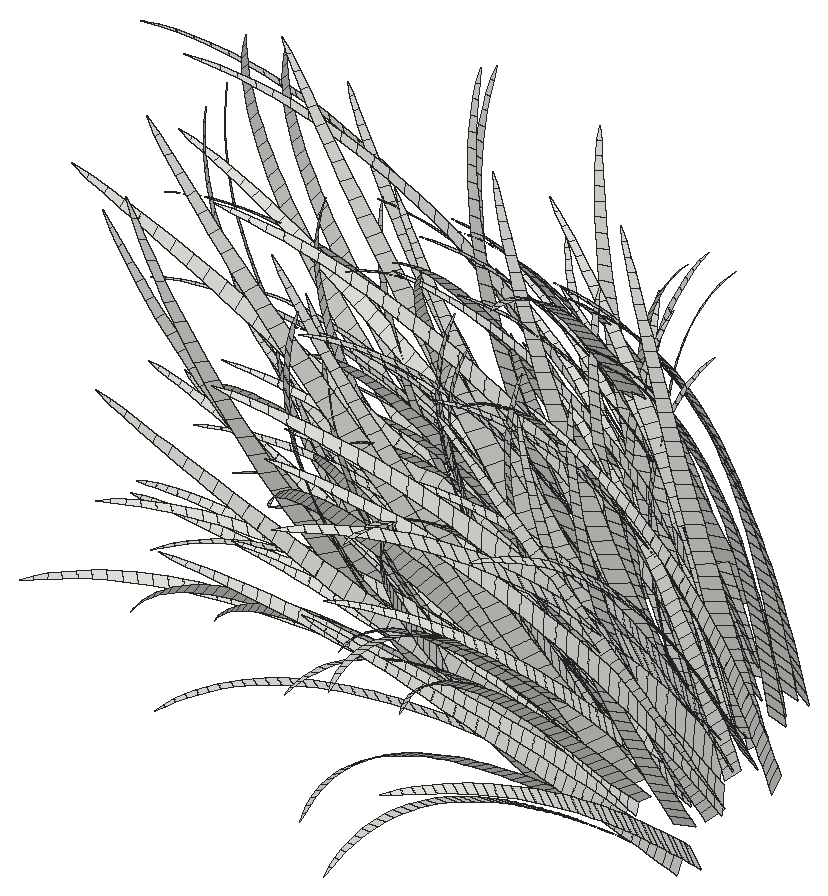
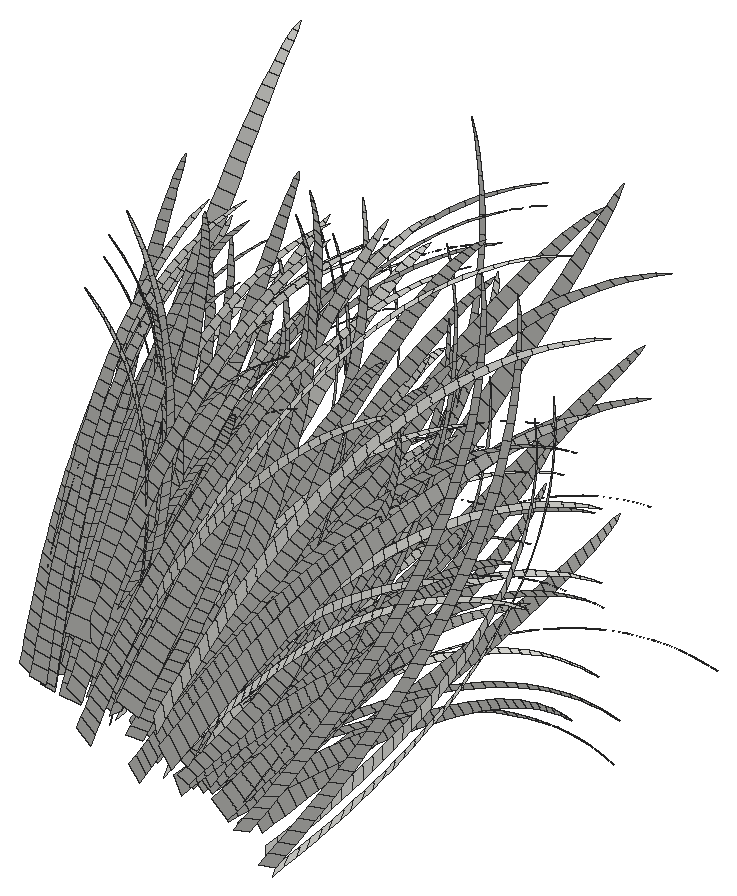
# SketchUp Ruby script. Lengths in inches.
U = 1.inch
M = Sketchup.active_model
def pt(a) = Geom::Point3d.new(a.map { |v| v * U })
def face(e, loops, mat)
  f = e.add_face(loops[0].map { |a| pt(a) })
  loops[1..].each { |l| e.add_face(l.map { |a| pt(a) }).erase! }
  f.material = f.back_material = mat if mat
  f
end
# faces: each face lists its corners as indices into pts; further lists are holes
def faces(e, pts, list, mat = nil) = list.each { |f| face(e, (f[0].is_a?(Array) ? f : [f]).map { |l| l.map { |i| pts[i] } }, mat) }
# xy, xz, yz: faces in a plane at the given z, y or x. An outline is a flat list of corners, or four numbers for a rectangle; further outlines are holes
def ring(l) = l.size == 4 ? [[l[0], l[1]], [l[2], l[1]], [l[2], l[3]], [l[0], l[3]]] : l.each_slice(2).to_a
def flat(e, list, mat, &to3) = list.each { |f| face(e, (f[0].is_a?(Array) ? f : [f]).map { |l| ring(l).map { |u, v| to3.(u, v) } }, mat) }
def xy(e, z, list, mat = nil) = flat(e, list, mat) { |x, y| [x, y, z] }
def xz(e, y, list, mat = nil) = flat(e, list, mat) { |x, z| [x, y, z] }
def yz(e, x, list, mat = nil) = flat(e, list, mat) { |y, z| [x, y, z] }
def lines(e, pts, list) = list.each { |a, b| e.add_line(pt(pts[a]), pt(pts[b])) }
# prism: a flat outline (further loops are holes) pulled along v
def prism(e, loops, v, mat = nil)
  f = face(e, loops, mat); d = Geom::Vector3d.new(v.map { |x| x * U })
  f.pushpull(f.normal.samedirection?(d) ? d.length : -d.length)
end
def box(e, o, s, mat = nil) = prism(e, [[o, [o[0] + s[0], o[1], o[2]], [o[0] + s[0], o[1] + s[1], o[2]], [o[0], o[1] + s[1], o[2]]]], [0, 0, s[2]], mat)
def at(x, y, z, deg = 0) = Geom::Transformation.translation(pt([x, y, z])) * Geom::Transformation.rotation(ORIGIN, Z_AXIS, deg.degrees)
def axes(o, x, y, z) = Geom::Transformation.new([*x, 0, *y, 0, *z, 0, *pt(o).to_a, 1])
def part(name) = M.definitions.add(name)
# library, detail: a bought-in or finely detailed component or shape, given as its bounding box
def library(name, o, s) = part(name).tap { |d| box(d.entities, o, s) }
def detail(e, o, s) = box(e.add_group.entities, o, s)
def put(e, d, t, mat = nil) = e.add_instance(d, t).tap { |i| i.material = mat if mat }
def group(e, t, mat = nil) = e.add_group.tap { |g| g.transformation = t; g.material = mat if mat }.entities
root = M.entities
c1 = part("fur_instance\#8")
p = [[-0.25,1.49,0.03],[0.25,-1.49,-0.03],[0.44,-1.47,1.51],[-0.05,1.47,1.57],[0.65,-1.44,3.05],[0.16,1.45,3.11],
  [0.86,-1.42,4.59],[0.38,1.44,4.65],[1.1,-1.39,6.13],[0.62,1.43,6.18],[1.34,-1.35,7.66],[0.875,1.42,7.72],
  [1.6,-1.32,9.19],[1.14,1.41,9.25],[1.88,-1.28,10.72],[1.43,1.41,10.78],[2.18,-1.24,12.25],[1.73,1.41,12.3],
  [2.49,-1.19,13.77],[2.05,1.41,13.82],[2.83,-1.15,15.29],[2.4,1.41,15.34],[3.18,-1.09,16.8],[2.76,1.42,16.85],
  [3.56,-1.03,18.31],[3.14,1.43,18.35],[3.96,-0.97,19.81],[3.55,1.44,19.85],[4.38,-0.91,21.3],[3.99,1.46,21.35],
  [4.84,-0.83,22.78],[4.45,1.48,22.83],[5.32,-0.76,24.26],[4.93,1.51,24.31],[5.82,-0.67,25.73],[5.45,1.54,25.77],
  [6.36,-0.59,27.18],[6,1.57,27.23],[6.93,-0.49,28.625],[6.58,1.61,28.67],[7.54,-0.39,30.05],[7.19,1.66,30.1],
  [8.18,-0.28,31.47],[7.84,1.71,31.51],[8.85,-0.16,32.86],[8.53,1.77,32.9],[9.57,-0.04,34.24],[9.25,1.83,34.27],
  [10.32,0.09,35.59],[10.02,1.9,35.625],[11.12,0.23,36.92],[10.82,1.97,36.95],[11.95,0.38,38.22],[11.67,2.06,38.25],
  [12.84,0.54,39.49],[12.57,2.14,39.52],[13.76,0.71,40.73],[13.51,2.24,40.76],[14.73,0.89,41.93],[14.49,2.34,41.95],
  [15.75,1.08,43.09],[15.52,2.45,43.11],[16.82,1.28,44.2],[16.6,2.5625,44.23],[17.93,1.5,45.27],[17.73,2.68,45.29],
  [19.08,1.73,46.28],[18.9,2.81,46.3],[20.29,1.97,47.24],[20.125,2.93,47.26],[21.53,2.22,48.13],[21.39,3.0625,48.15],
  [22.82,2.5,48.96],[22.7,3.1875,48.98],[24.14,2.8125,49.72],[24.06,3.3,49.73],[25.48,3.27,50.41]]
faces(c1.entities,p,[[0,1,2,3],[3,2,4,5],[5,4,6,7],[7,6,8,9],[9,8,10,11],[11,10,12,13],[13,12,14,15],[15,14,16,17],
  [17,16,18,19],[19,18,20,21],[21,20,22,23],[23,22,24,25],[25,24,26,27],[27,26,28,29],[29,28,30,31],[31,30,32,33],
  [33,32,34,35],[35,34,36,37],[37,36,38,39],[39,38,40,41],[41,40,42,43],[43,42,44,45],[45,44,46,47],[47,46,48,49],
  [49,48,50,51],[51,50,52,53],[53,52,54,55],[55,54,56,57],[57,56,58,59],[59,58,60,61],[61,60,62,63],[63,62,64,65],
  [65,64,66,67],[67,66,68,69],[69,68,70,71],[71,70,72,73],[73,72,74,75],[75,74,76]])
put(root,c1,axes([286.59,30.47,9.65],[0.27343,-0.05373,0.34841],[-0.11723,0.29702,0.06467],[-0.32726,-0.11352,0.28294]))
put(root,c1,axes([287.23,30.26,10.09],[0.23007,0.02662,0.34929],[-0.18351,0.2974,-0.02967],[-0.32374,-0.1123,0.27989]))
put(root,c1,axes([285.25,32.66,11.29],[0.334,-0.2152,0.2493],[0.13177,0.25584,0.18399],[-0.3051,-0.07912,0.37064]))
put(root,c1,axes([291.09,32.8125,16.03],[-0.40111,-0.111,-0.15079],[0.2354,-0.31959,0.01115],[-0.14507,-0.1083,0.47608]))
put(root,c1,axes([291.52,27.75,9.48],[-0.20253,0.22492,-0.01123],[-0.17196,-0.03802,-0.28818],[-0.24112,-0.12808,0.22836]))
put(root,c1,axes([292.69,26.93,10.13],[-0.26498,0.16022,-0.17783],[-0.02095,-0.16252,-0.22723],[-0.24124,-0.12814,0.22846]))
put(root,c1,axes([287.03,32.11,12.13],[0.3301,-0.20151,0.24919],[0.11757,0.2566,0.17128],[-0.29775,-0.07722,0.36172]))
put(root,c1,axes([291.21,31.99,14.07],[-0.17529,-0.2316,-0.142],[0.33875,-0.20497,0.16137],[-0.21428,-0.07814,0.39369]))
put(root,c1,axes([292.88,25.97,10.52],[-0.32801,0.05137,-0.26925],[0.18585,-0.20887,-0.21385],[-0.19763,-0.22375,0.26878]))
put(root,c1,axes([292.88,26.65,9.85],[-0.28984,0.15344,-0.12784],[-0.02507,-0.13644,-0.25763],[-0.20658,-0.15978,0.2261]))
put(root,c1,axes([293.18,28.9,13.9],[-0.37766,0.184,-0.06914],[-0.15358,-0.20823,-0.20885],[-0.16081,-0.1578,0.39181]))
put(root,c1,axes([292.93,26.43,10.32],[-0.31045,0.17685,-0.06933],[-0.11896,-0.14445,-0.24345],[-0.18306,-0.15633,0.29554]))
put(root,c1,axes([292.82,29.91,11.98],[-0.30983,-0.00394,-0.17456],[0.06503,-0.26267,0.03289],[-0.18102,-0.0412,0.32902]))
put(root,c1,axes([292.9,29.58,13.37],[-0.30671,-0.07302,-0.20131],[0.19117,-0.27097,0.01937],[-0.18997,-0.09935,0.36653]))
put(root,c1,axes([291.91,26.05,10.63],[-0.20515,0.19921,0.286],[-0.39464,0.04212,-0.25253],[-0.15677,-0.2771,0.29704]))
put(root,c1,axes([290.35,29.43,10.8],[0.11044,-0.26664,-0.03562],[0.2879,-0.01439,0.25595],[-0.24023,-0.09964,0.30634]))
put(root,c1,axes([293.35,26.83,10.48],[-0.21721,0.20602,0.03558],[-0.22128,-0.05396,-0.23339],[-0.17073,-0.1458,0.27564]))
put(root,c1,axes([294.49,26.96,13.81],[-0.4809,0.15467,0.07003],[-0.17758,-0.1848,-0.34168],[-0.0839,-0.29221,0.4025]))
put(root,c1,axes([292.82,27.34,10.21],[-0.12157,0.22306,0.06553],[-0.25945,0.01126,-0.21995],[-0.19306,-0.11653,0.26984]))
put(root,c1,axes([290.16,27.27,9.43],[0.16873,-0.23329,-0.16268],[0.2954,-0.05676,0.29434],[-0.24156,-0.18683,0.26439]))
put(root,c1,axes([294.54,30.98,16.64],[-0.45841,-0.0448,-0.1227],[0.16046,-0.32039,-0.10023],[-0.09604,-0.16019,0.48225]))
put(root,c1,axes([293.29,28.56,10.54],[-0.11106,-0.1633,-0.14192],[0.22222,-0.16383,0.16068],[-0.2111,-0.05474,0.25645]))
put(root,c1,axes([294.5,25.83,11.2],[-0.36489,0.00046,-0.19285],[0.17529,-0.2126,-0.2068],[-0.11798,-0.22209,0.32702]))
put(root,c1,axes([293.99,26.59,11.08],[-0.20712,-0.07699,-0.24552],[0.24774,-0.208,-0.01302],[-0.1778,-0.15184,0.28705]))
put(root,c1,axes([293.27,28.91,13.42],[-0.15645,0.26226,0.09015],[-0.35289,-0.02097,-0.18778],[-0.15226,-0.14941,0.37098]))
put(root,c1,axes([294.61,29.11,11.65],[-0.25641,-0.05967,-0.14526],[0.12307,-0.22834,0.06607],[-0.16263,-0.03702,0.2956]))
put(root,c1,axes([293.88,25.64,11.62],[-0.31647,0.23033,0.24139],[-0.40723,-0.07569,-0.25469],[-0.08441,-0.29398,0.40494]))
put(root,c1,axes([290.57,27.84,9.43],[0.27393,-0.09989,0.26383],[-0.07841,0.22332,0.16142],[-0.25859,-0.13736,0.2449]))
put(root,c1,axes([294.43,26.1,10.01],[-0.20297,0.18888,0.02954],[-0.20068,-0.0525,-0.2153],[-0.15716,-0.13421,0.25373]))
put(root,c1,axes([294,25.73,9.63],[-0.1796,-0.03718,-0.28054],[0.25918,-0.17602,-0.0633],[-0.1653,-0.18714,0.2248]))
put(root,c1,axes([295.09,25.85,10.55],[-0.31089,0.06016,-0.13906],[0.05838,-0.17982,-0.18276],[-0.13322,-0.16333,0.26664]))
put(root,c1,axes([289.54,28.61,11.13],[0.35824,-0.10563,0.23396],[-0.03698,0.2601,0.16876],[-0.24267,-0.14648,0.33917]))
put(root,c1,axes([292.97,24.9375,9.61],[-0.15927,0.19141,0.39707],[-0.5038,0.04411,-0.1792],[-0.10137,-0.33957,0.3384]))
put(root,c1,axes([295.47,24.97,10.55],[-0.40671,0.13906,0.11983],[-0.19446,-0.09353,-0.35183],[-0.08649,-0.28972,0.28872]))
put(root,c1,axes([292.35,27.91,11],[0.09607,0.16636,0.21346],[-0.29279,0.17326,-0.12392],[-0.20763,-0.12533,0.2902]))
put(root,c1,axes([294.18,27.19,13.6],[-0.24749,0.26545,0.14907],[-0.39506,-0.07422,-0.19021],[-0.10328,-0.2127,0.42576]))
put(root,c1,axes([294.73,26.92,12.03],[-0.31144,-0.04433,-0.1638],[0.17873,-0.22297,-0.09563],[-0.11163,-0.15329,0.33567]))
put(root,c1,axes([294.97,26.6,11.01],[-0.16359,0.19718,0.06974],[-0.23715,-0.01659,-0.20797],[-0.15863,-0.13546,0.2561]))
put(root,c1,axes([294.36,30.1,11.41],[-0.13255,-0.19412,-0.04324],[0.25386,-0.13806,0.15203],[-0.15874,-0.01602,0.29618]))
put(root,c1,axes([293.23,27.37,10.11],[0.05622,-0.22028,-0.06146],[0.25349,-0.04511,0.20874],[-0.20228,-0.0839,0.25794]))
put(root,c1,axes([291.99,26.66,9.55],[0.19826,-0.21945,-0.10113],[0.24048,-0.01499,0.29104],[-0.22131,-0.17117,0.24222]))
put(root,c1,axes([295.96,26.78,12.57],[-0.37408,0.03214,-0.09204],[0.05374,-0.22112,-0.17294],[-0.08373,-0.17243,0.34515]))
put(root,c1,axes([292.83,28.6,10.86],[0.14214,-0.23634,0.06971],[0.22005,0.06034,0.21505],[-0.2226,-0.05773,0.27043]))
put(root,c1,axes([292.76,29.2,12.34],[0.06163,-0.26061,-0.05185],[0.33201,-0.02894,0.18171],[-0.1775,-0.09282,0.34246]))
put(root,c1,axes([296.13,24.84,10.15],[-0.38075,0.07768,-0.02207],[-0.01808,-0.11852,-0.3135],[-0.07313,-0.24497,0.24413]))
put(root,c1,axes([295.55,28.38,12.91],[-0.29669,-0.08119,-0.1125],[0.1791,-0.23152,-0.01214],[-0.09804,-0.09366,0.35151]))
put(root,c1,axes([294.97,25.4,9.79],[-0.08632,0.15484,0.21721],[-0.29175,0.07846,-0.1727],[-0.1595,-0.18058,0.21691]))
put(root,c1,axes([296.28,30.79,13.71],[-0.31442,-0.10008,-0.0717],[0.17027,-0.25235,0.08233],[-0.10906,-0.0245,0.3674]))
put(root,c1,axes([294.48,28.84,11.72],[-0.04846,-0.21474,-0.06537],[0.28534,-0.09466,0.14944],[-0.1626,-0.0593,0.29875]))
put(root,c1,axes([296.46,25.04,10.21],[-0.31964,0.05744,-0.08852],[0.03295,-0.15868,-0.20626],[-0.09365,-0.17629,0.25958]))
put(root,c1,axes([296.53,26.36,11.67],[-0.31367,0.05166,-0.09146],[0.01951,-0.19214,-0.13854],[-0.0977,-0.13416,0.29378]))
put(root,c1,axes([294.97,28.29,12.09],[-0.06107,-0.20437,-0.10373],[0.29349,-0.11146,0.13184],[-0.15758,-0.08241,0.30403]))
put(root,c1,axes([292.65,27.21,10.55],[0.22564,-0.22209,0.02694],[0.20271,0.08113,0.24146],[-0.20438,-0.12337,0.28566]))
put(root,c1,axes([295.73,27.23,12.77],[-0.1569,0.2286,0.10904],[-0.32818,-0.02785,-0.15821],[-0.11309,-0.15528,0.34003]))
put(root,c1,axes([297.22,28.28,15.37],[-0.48448,0.00048,-0.04012],[0.07209,-0.2662,-0.24534],[-0.01781,-0.23845,0.43674]))
put(root,c1,axes([293.88,25.5,9.7],[0.14772,0.06981,0.31071],[-0.30774,0.18182,0.01975],[-0.17895,-0.2026,0.24337]))
put(root,c1,axes([296.17,25.125,10.97],[-0.24536,0.19524,0.21246],[-0.35336,-0.05273,-0.20133],[-0.07041,-0.24522,0.33777]))
put(root,c1,axes([295.57,27.91,12.12],[-0.06025,-0.19978,-0.10172],[0.28707,-0.10941,0.12883],[-0.15419,-0.08063,0.29748]))
put(root,c1,axes([291.96,26.95,11.7],[0.27785,-0.24567,-0.11356],[0.31431,0.05376,0.28262],[-0.17668,-0.21661,0.35363]))
put(root,c1,axes([293.34,28.62,13.62],[0.18292,0.18783,0.21033],[-0.35625,0.19804,-0.04959],[-0.15796,-0.15501,0.38486]))
put(root,c1,axes([295.89,31.56,13.24],[-0.16074,-0.22509,0.01009],[0.31616,-0.14511,0.10525],[-0.09686,-0.01193,0.36183]))
put(root,c1,axes([292.11,29.1,12.95],[0.32177,-0.21274,0.07133],[0.19821,0.17649,0.19557],[-0.17683,-0.12709,0.37373]))
put(root,c1,axes([291.88,25.43,9.8],[0.36191,0.00675,0.33836],[-0.31641,0.21997,0.23571],[-0.16944,-0.29949,0.32104]))
put(root,c1,axes([294.33,27.9,13.69],[0.10522,0.22276,0.21396],[-0.40669,0.14528,-0.0588],[-0.1306,-0.17932,0.39268]))
put(root,c1,axes([295.03,27.92,12.46],[0.04713,-0.23319,-0.08917],[0.32063,-0.04249,0.15465],[-0.15163,-0.10898,0.32048]))
put(root,c1,axes([295.61,30.37,15.29],[-0.09495,-0.26399,-0.12104],[0.41267,-0.12196,0.06705],[-0.10338,-0.12826,0.42496]))
put(root,c1,axes([294.625,30.24,14.41],[0.02749,-0.28529,-0.04854],[0.39441,-0.03638,0.11901],[-0.12332,-0.09206,0.40471]))
put(root,c1,axes([293.7,27.38,10.89],[0.2739,-0.05108,0.20185],[-0.0714,0.21464,0.10324],[-0.19072,-0.11512,0.26657]))
put(root,c1,axes([296.78,27.66,13.94],[-0.30159,-0.14954,-0.10961],[0.28485,-0.21676,-0.0779],[-0.03755,-0.15132,0.40536]))
put(root,c1,axes([295.99,25.24,10.68],[-0.01763,-0.16784,-0.246],[0.36343,-0.09136,0.06391],[-0.10604,-0.19963,0.29394]))
put(root,c1,axes([293.74,26.66,11.29],[0.29218,0.02035,0.226],[-0.20172,0.21186,0.12397],[-0.14953,-0.18332,0.29929]))
put(root,c1,axes([298.23,27.93,12.79],[-0.30076,0.11654,-0.01023],[-0.13091,-0.19765,-0.03854],[-0.03233,-0.07151,0.33559]))
put(root,c1,axes([295.5,25.92,10.87],[0.0874,-0.18327,-0.1671],[0.30131,-0.04217,0.15478],[-0.13212,-0.16199,0.26446]))
put(root,c1,axes([297.23,28.02,12.74],[-0.08042,0.22658,0.04044],[-0.31016,-0.01086,-0.09649],[-0.09064,-0.0866,0.32499]))
put(root,c1,axes([297.87,30.0625,14.61],[-0.28554,-0.16794,-0.04721],[0.27744,-0.2201,-0.01414],[-0.03336,-0.09063,0.40665]))
put(root,c1,axes([297.125,30.625,14.38],[-0.18942,-0.22658,-0.02013],[0.33953,-0.1634,0.03397],[-0.04803,-0.05962,0.39971]))
put(root,c1,axes([295.45,28.78,12.12],[0.18989,-0.20261,0.10406],[0.21185,0.12115,0.12104],[-0.16267,-0.03703,0.29567]))
put(root,c1,axes([295.74,24.72,9.42],[0.0858,-0.14547,-0.26588],[0.34076,-0.06868,0.14201],[-0.12385,-0.21892,0.23467]))
put(root,c1,axes([294.01,26.75,11.5],[0.32008,-0.01898,0.19642],[-0.14214,0.20908,0.16147],[-0.14749,-0.18083,0.29522]))
put(root,c1,axes([298.91,28.66,14.45],[-0.38324,-0.06278,-0.0243],[0.13399,-0.24652,-0.1286],[0.00956,-0.15154,0.39527]))
put(root,c1,axes([298.92,28.0625,13.11],[-0.32632,0.09549,0.01183],[-0.10602,-0.21576,-0.04162],[-0.01005,-0.0835,0.34927]))
put(root,c1,axes([299.78,25.77,12.74],[-0.51625,-0.01769,0.01101],[0.05539,-0.22677,-0.34952],[0.04511,-0.30441,0.40404]))
put(root,c1,axes([298.68,25.23,11.32],[-0.31274,-0.0305,-0.0904],[0.13256,-0.1462,-0.20962],[-0.01285,-0.1978,0.26335]))
put(root,c1,axes([299.29,24.02,9.18],[-0.33771,0.05415,0.06448],[-0.07902,-0.09732,-0.27357],[-0.01313,-0.22725,0.21826]))
put(root,c1,axes([293.32,25.6,9.97],[0.3863,-0.08495,0.14429],[-0.0772,0.15908,0.30557],[-0.13885,-0.24542,0.26308]))
put(root,c1,axes([295.53,25.8,11.74],[0.07034,-0.19682,-0.2749],[0.41946,-0.0352,0.0904],[-0.06961,-0.24244,0.33395]))
put(root,c1,axes([296.12,26.47,13],[0.01216,-0.24161,-0.22015],[0.43971,-0.04869,0.04603],[-0.05692,-0.2094,0.39526]))
put(root,c1,axes([297.77,26.32,12.95],[-0.12746,0.22793,0.20456],[-0.40492,-0.03571,-0.06764],[-0.01543,-0.20666,0.37851]))
put(root,c1,axes([300.32,25.23,11.71],[-0.46527,-0.01659,0.00893],[0.0514,-0.2044,-0.31514],[0.04067,-0.27444,0.36426]))
put(root,c1,axes([297.48,28.18,12.65],[-0.09581,-0.20834,-0.02839],[0.30832,-0.09424,0.02399],[-0.03855,-0.06264,0.3313]))
put(root,c1,axes([297.57,24.18,9.17],[-0.04371,-0.10656,-0.29777],[0.35851,-0.08169,-0.00106],[-0.06929,-0.23211,0.23131]))
put(root,c1,axes([299.37,26.42,13.65],[-0.38898,-0.12138,-0.1563],[0.28848,-0.17401,-0.28627],[0.04207,-0.28393,0.37685]))
put(root,c1,axes([297.625,27.6,13.88],[-0.04344,0.25829,0.12602],[-0.405,0.01192,-0.03938],[-0.03687,-0.14857,0.39801]))
put(root,c1,axes([298.99,28.8,14.17],[-0.26677,-0.17563,-0.03118],[0.2823,-0.20104,-0.03743],[-0.00389,-0.09462,0.39526]))
put(root,c1,axes([296.59,25.125,10.45],[0.12474,-0.17137,-0.17547],[0.30213,-0.01003,0.14608],[-0.09526,-0.17933,0.26405]))
put(root,c1,axes([299.73,26.4,12.67],[-0.33399,-0.07506,-0.0555],[0.16081,-0.18656,-0.17968],[0.02085,-0.18123,0.33096]))
put(root,c1,axes([299.39,27.85,13.625],[-0.27779,-0.14446,-0.06814],[0.25565,-0.18732,-0.10083],[0.00889,-0.14091,0.36755]))
put(root,c1,axes([297.62,28.84,14.35],[-0.0089,-0.25066,-0.12068],[0.39466,-0.05132,0.04383],[-0.05759,-0.13838,0.38836]))
put(root,c1,axes([296.65,25.52,11.22],[0.21687,0.07669,0.22313],[-0.26692,0.16353,0.08902],[-0.10023,-0.18868,0.27783]))
put(root,c1,axes([297.63,30.28,13.83],[-0.01692,-0.26276,0.01097],[0.36797,-0.04078,0.03189],[-0.03963,-0.04761,0.37835]))
put(root,c1,axes([299.97,26.26,12.16],[-0.29317,0.10093,0.07385],[-0.14377,-0.18016,-0.07471],[0.02576,-0.11996,0.31897]))
put(root,c1,axes([300.07,27.16,13.45],[-0.29271,0.17428,0.10924],[-0.25994,-0.17585,-0.06269],[0.03088,-0.14382,0.38241]))
put(root,c1,axes([300.13,25.01,11.1],[-0.28203,0.10587,0.18201],[-0.23358,-0.12053,-0.16644],[0.03181,-0.2147,0.28497]))
put(root,c1,axes([300.1,27.49,12.94],[-0.30393,0.1052,0.0905],[-0.15495,-0.19294,-0.06173],[0.04464,-0.12101,0.33532]))
put(root,c1,axes([295.98,29.34,13.36],[0.34293,-0.08305,0.10265],[0.05105,0.24395,0.04412],[-0.11421,-0.06659,0.35721]))
put(root,c1,axes([299.87,24.17,9.58],[-0.27633,-0.0611,-0.12055],[0.1825,-0.08553,-0.24132],[0.03785,-0.21912,0.20981]))
put(root,c1,axes([296.4,29.08,12.81],[0.31176,0.0256,0.10043],[-0.08475,0.24227,-0.02143],[-0.10796,-0.04837,0.33382]))
put(root,c1,axes([298.25,26.49,12.56],[0.05887,0.18099,0.17896],[-0.34505,0.07557,-0.00169],[-0.0453,-0.16663,0.31453]))
put(root,c1,axes([297.05,26.73,12.2],[0.1871,0.14964,0.10604],[-0.26661,0.15708,0.00666],[-0.06441,-0.10742,0.32341]))
put(root,c1,axes([298.57,27.15,12.59],[0.01132,0.20294,0.10412],[-0.32522,0.03856,-0.01693],[-0.02945,-0.1187,0.31798]))
put(root,c1,axes([299,24.64,10.45],[-0.04666,0.14964,0.22675],[-0.3377,0.00868,-0.03278],[-0.0129,-0.19852,0.26431]))
put(root,c1,axes([296.7,28.29,13.21],[0.27868,0.10232,0.11206],[-0.21064,0.21699,0.02173],[-0.08528,-0.10581,0.35058]))
put(root,c1,axes([300.49,29.72,14.09],[-0.26519,-0.17991,0.01243],[0.275,-0.19993,-0.03913],[0.02658,-0.07504,0.39049]))
put(root,c1,axes([297.26,30.11,16.83],[0.06158,-0.31848,-0.16233],[0.50389,0.0002,0.02365],[-0.01699,-0.18902,0.49426]))
put(root,c1,axes([299.67,29.26,13.5],[-0.16387,-0.2151,0.01341],[0.31522,-0.13246,-0.03206],[0.02509,-0.06018,0.3635]))
put(root,c1,axes([299.65,29.91,13.88],[-0.15998,-0.22934,0.01844],[0.33411,-0.13168,-0.02904],[0.02425,-0.05773,0.37906]))
put(root,c1,axes([299.76,29.12,13.14],[-0.14664,-0.21176,0.02108],[0.30791,-0.12172,-0.02142],[0.01937,-0.04876,0.34894]))
put(root,c1,axes([299.19,25.09,11.2],[0.03575,0.14554,0.23167],[-0.3445,0.04481,0.02258],[-0.01311,-0.20168,0.26852]))
put(root,c1,axes([297.38,27.1,12.38],[0.28278,0.06506,0.09164],[-0.15628,0.20514,0.05207],[-0.06389,-0.10656,0.32081]))
put(root,c1,axes([300.24,27.14,13.48],[-0.16291,0.19785,0.19896],[-0.35679,-0.09309,-0.02257],[0.05771,-0.18908,0.35373]))
put(root,c1,axes([300.45,26.58,12.89],[-0.22027,-0.1762,-0.1173],[0.31356,-0.12079,-0.15656],[0.05639,-0.18473,0.34559]))
put(root,c1,axes([301.79,26.51,12.29],[-0.34984,0.00375,0.09918],[-0.0319,-0.20604,-0.15196],[0.08245,-0.16358,0.32241]))
